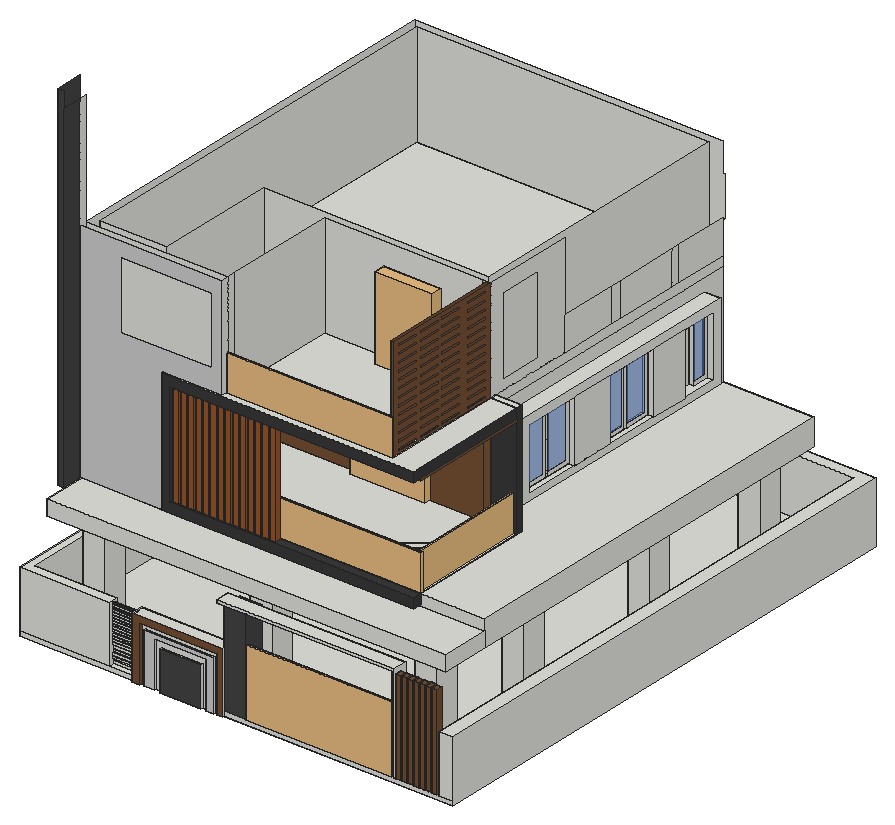
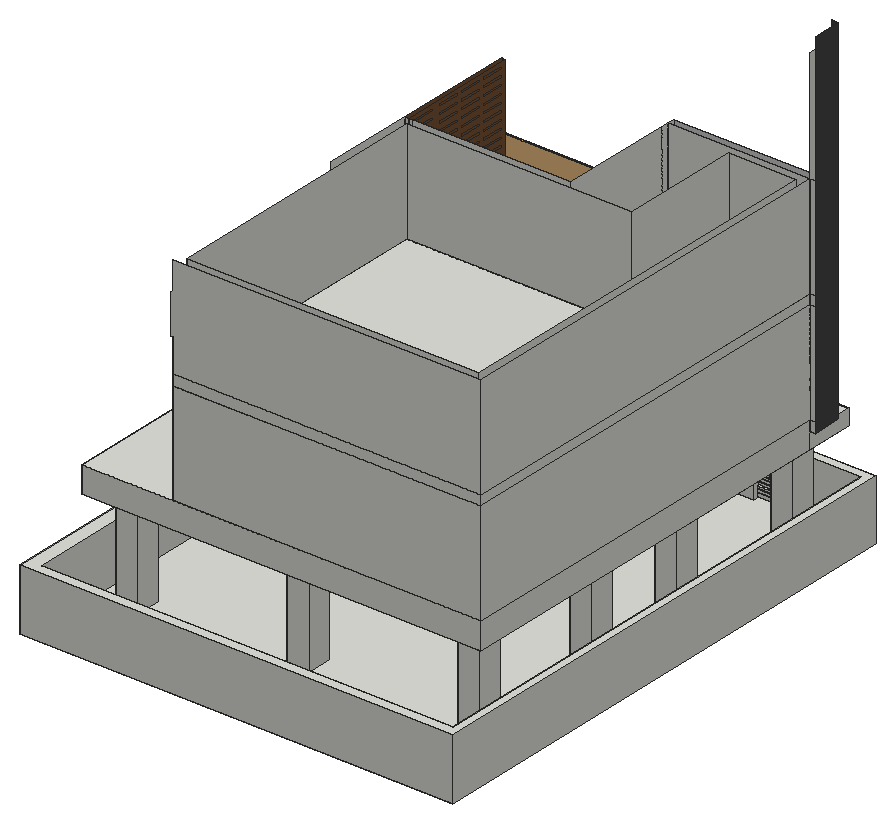
# SketchUp Ruby script. Lengths in inches.
U = 1.inch
M = Sketchup.active_model
def pt(a) = Geom::Point3d.new(a.map { |v| v * U })
def face(e, loops, mat)
  f = e.add_face(loops[0].map { |a| pt(a) })
  loops[1..].each { |l| e.add_face(l.map { |a| pt(a) }).erase! }
  f.material = f.back_material = mat if mat
  f
end
# faces: each face lists its corners as indices into pts; further lists are holes
def faces(e, pts, list, mat = nil) = list.each { |f| face(e, (f[0].is_a?(Array) ? f : [f]).map { |l| l.map { |i| pts[i] } }, mat) }
# xy, xz, yz: faces in a plane at the given z, y or x. An outline is a flat list of corners, or four numbers for a rectangle; further outlines are holes
def ring(l) = l.size == 4 ? [[l[0], l[1]], [l[2], l[1]], [l[2], l[3]], [l[0], l[3]]] : l.each_slice(2).to_a
def flat(e, list, mat, &to3) = list.each { |f| face(e, (f[0].is_a?(Array) ? f : [f]).map { |l| ring(l).map { |u, v| to3.(u, v) } }, mat) }
def xy(e, z, list, mat = nil) = flat(e, list, mat) { |x, y| [x, y, z] }
def xz(e, y, list, mat = nil) = flat(e, list, mat) { |x, z| [x, y, z] }
def yz(e, x, list, mat = nil) = flat(e, list, mat) { |y, z| [x, y, z] }
def lines(e, pts, list) = list.each { |a, b| e.add_line(pt(pts[a]), pt(pts[b])) }
# prism: a flat outline (further loops are holes) pulled along v
def prism(e, loops, v, mat = nil)
  f = face(e, loops, mat); d = Geom::Vector3d.new(v.map { |x| x * U })
  f.pushpull(f.normal.samedirection?(d) ? d.length : -d.length)
end
def box(e, o, s, mat = nil) = prism(e, [[o, [o[0] + s[0], o[1], o[2]], [o[0] + s[0], o[1] + s[1], o[2]], [o[0], o[1] + s[1], o[2]]]], [0, 0, s[2]], mat)
def at(x, y, z, deg = 0) = Geom::Transformation.translation(pt([x, y, z])) * Geom::Transformation.rotation(ORIGIN, Z_AXIS, deg.degrees)
def axes(o, x, y, z) = Geom::Transformation.new([*x, 0, *y, 0, *z, 0, *pt(o).to_a, 1])
def part(name) = M.definitions.add(name)
# library, detail: a bought-in or finely detailed component or shape, given as its bounding box
def library(name, o, s) = part(name).tap { |d| box(d.entities, o, s) }
def detail(e, o, s) = box(e.add_group.entities, o, s)
def put(e, d, t, mat = nil) = e.add_instance(d, t).tap { |i| i.material = mat if mat }
def group(e, t, mat = nil) = e.add_group.tap { |g| g.transformation = t; g.material = mat if mat }.entities
root = M.entities
M.materials.add("[Carrera Marble]").color = [207, 207, 207]
M.materials.add("[Color M07]").color = [58, 58, 58]
M.materials.add("[Granite Dark Gray]").color = [69, 68, 68]
M.materials.add("[Sandstone]").color = [118, 81, 52]
M.materials.add("[Translucent Glass Blue]").color = [100, 149, 237]
M.materials["[Translucent Glass Blue]"].alpha = 0.5
M.materials.add("[Wood Cherry Original]").color = [152, 86, 42]
c1 = part("Group\#1")
box(c1.entities,[0,-120,0],[26.125,120,28.5])
c2 = library("Modern Gate 1",[0,0,0],[118.11,1.97,78.74])
c3 = part("Group\#42")
box(c3.entities,[-2.625,0,0],[5.625,7.625,109.5625])
c4 = library("Wagner Glass Railing",[9.08,102.375,1.53],[2.51,145.5,42.05])
c5 = library("Glazed double door",[0,0,0],[62.99,7.48,78.74])
c6 = part("Group\#2")
box(c6.entities,[0,0,0],[7.1875,5.875,122.9375],"[Wood Cherry Original]")
c7 = part("Janela aluminio\#1")
xy(c7.entities,0,[[0,0,47.24,1.57],[23.62,1.57,47.24,2.76],[0,2.76,25.98,3.9375],[0,3.9375,47.24,5.91]])
xy(c7.entities,43.31,[[0,0,47.24,1.57],[23.62,1.57,47.24,2.76],[0,2.76,0,5.91,47.24,5.91,47.24,3.9375,25.98,3.9375,25.98,2.76],[25.98,2.76,47.24,3.9375]])
xz(c7.entities,1.57,[[0,0,23.62,0,23.62,41.34,21.26,41.34,21.26,1.97,1.97,1.97,1.97,41.34,23.62,41.34,23.62,43.31,0,43.31],[[23.62,0,47.24,43.31],[25.7,1.97,45.28,41.34]]])
xz(c7.entities,2.76,[[[0,0,23.62,43.31],[2.36,2.36,21.26,40.94]],[23.62,0,25.98,43.31]])
xz(c7.entities,2.76,[[2.36,2.36,21.26,40.94]],"[Translucent Glass Blue]")
xz(c7.entities,3.9375,[[25.98,0,25.98,2.36,44.88,2.36,44.88,40.94,25.98,40.94,25.98,43.31,47.24,43.31,47.24,0]])
xz(c7.entities,3.9375,[[25.98,2.36,44.88,40.94]],"[Translucent Glass Blue]")
yz(c7.entities,0,[[0,0,1.57,43.31],[2.76,0,5.91,43.31]])
yz(c7.entities,23.62,[[1.57,0,2.76,43.31]])
yz(c7.entities,25.98,[[2.76,0,3.9375,43.31]])
yz(c7.entities,47.24,[[0,0,1.57,43.31],[1.57,0,2.76,43.31],[3.9375,0,5.91,43.31]])
c8 = part("Group\#5")
prism(c8.entities,[[[0,0,131.51],[0,0,140.51],[8.96,0,140.51],[21.98,0,140.51],[21.98,0,0],[0,0,0]]],[0,-2.3125,0])
c9 = part("Group\#4")
box(c9.entities,[0,-480,0],[360,480,12])
c10 = library("test",[125.61,35.04,0],[12.99,66.93,96.46])
box(root,[18.76,18.85,-141.29],[466.13,57.13,17.95])
xy(root,-266.29,[[147.24,0,147.24,2.375,0,2.375,0,620.47,505.875,620.47,505.875,2.375,228.33,2.375,228.33,0,219.08,0,219.08,2.375,213.55,2.375,213.55,0,165.63,0,165.63,2.375,159.24,2.375,159.24,0],[133.09,0,142.08,2.375],[231.94,0,238.97,2.375]])
xy(root,-261.29,[[104.9,2.375,133.09,2.375,133.09,14.25,238.97,14.25,238.97,25.4375,264.34,25.4375,264.34,2.375,434.35,2.375,434.35,18.875,437.54,18.875,437.54,2.375,489.68,2.375,489.68,608.34,9.22,608.34,9.22,13.4,104.9,13.4],[238.97,2.375,264.34,25.4375]])
xy(root,-259.28,[[104.9,6.59,134.72,9.9]])
xy(root,-255.96,[[104.9,6.59,134.72,9.9]])
xy(root,-254.51,[[104.9,6.36,135.03,9.73]])
xy(root,-251.88,[[104.9,6.36,135.03,9.73]])
xy(root,-250.74,[[104.9,6.31,135.47,9.43]])
xy(root,-248.3,[[104.9,6.31,135.47,9.43]])
xy(root,-247.03,[[104.9,6.39,135.03,8.95]])
xy(root,-244.47,[[104.9,6.39,135.03,8.95]])
xy(root,-243.26,[[104.9,6.39,135.22,8.51]])
xy(root,-240.82,[[104.9,6.39,135.22,8.51]])
xy(root,-239.6,[[104.9,6.24,136.03,8.49]])
xy(root,-237.35,[[104.9,6.24,136.03,8.49]])
xy(root,-236.07,[[104.9,5.99,134.59,8.24]])
xy(root,-234.01,[[104.9,5.99,134.59,8.24]])
xy(root,-232.8,[[104.9,5.84,136.53,8.09]])
xy(root,-230.92,[[104.9,5.84,136.53,8.09]])
xy(root,-229.72,[[104.9,5.97,142.08,8.41]])
xy(root,-227.65,[[104.9,5.97,142.08,8.41]])
xy(root,-225.66,[[104.9,5.73,135.78,8.17]])
xy(root,-223.91,[[104.9,5.73,135.78,8.17]])
xy(root,-222.46,[[104.9,5.5625,133.34,7.875]])
xy(root,-221.03,[[165.63,0,213.55,2.375]])
xy(root,-220.78,[[104.9,5.5625,133.34,7.875]])
xy(root,-219.6,[[104.9,5.51,142.08,7.82]])
xy(root,-217.97,[[104.9,5.51,142.08,7.82]])
xy(root,-216.74,[[104.9,5.42,138.72,7.61]])
xy(root,-215.12,[[104.9,5.42,138.72,7.61]])
xy(root,-213.64,[[104.9,5.39,135.9,7.45]])
xy(root,-212.45,[[159.24,0,219.08,2.375]])
xy(root,-212.01,[[104.9,5.39,135.9,7.45]])
xy(root,-210.69,[[104.9,5.36,134.65,7.36]])
xy(root,-208.69,[[104.9,5.36,134.65,7.36]])
xy(root,-207.6,[[147.24,0,228.33,2.375]])
xy(root,-207.35,[[104.9,5.15,136.84,6.9]])
xy(root,-205.6,[[104.9,5.15,136.84,6.9]])
xy(root,-204.41,[[104.9,5.07,136.15,6.88]])
xy(root,-202.6,[[104.9,5.07,136.15,6.88]])
xy(root,-202.06,[[142.08,0,231.94,2.375]],"[Sandstone]")
xy(root,-201.5,[[104.9,5.28,134.97,6.85]])
xy(root,-199.93,[[104.9,5.28,134.97,6.85]])
xy(root,-198.85,[[104.9,5.125,134.53,6.875]])
xy(root,-197.28,[[104.9,5.125,134.53,6.875]])
xy(root,-196.375,[[104.9,5.06,135.09,6.75]])
xy(root,-194.875,[[104.9,5.06,135.09,6.75]])
xy(root,-194.79,[[133.09,0,238.97,14.25]])
xy(root,-194.41,[[0,2.375,104.9,2.375,104.9,13.4,9.22,13.4,9.22,608.34,489.68,608.34,489.68,2.375,505.875,2.375,505.875,620.47,0,620.47]])
xy(root,-150.83,[[229.85,2.375,238.97,18.875],[238.97,2.375,264.34,18.875],[264.34,2.375,434.35,18.875],[238.97,18.875,264.34,25.4375]])
xy(root,-147.41,[[229.85,2.375,437.54,18.875]])
xy(root,-122.04,[[11.76,42.54,18.76,75.98],[115.14,65.73,115.14,75.98,379.07,75.98,379.07,224.17,409.51,224.17,409.51,65.73],[18.76,67.23,115.14,75.98]])
xy(root,-110.04,[[[18.76,75.98,18.76,555.98,378.76,555.98,378.76,216.49,115.14,216.49,115.14,75.98],[27.76,84.98,106.14,84.98,106.14,225.49,369.76,225.49,369.76,546.98,27.76,546.98]],[115.14,75.98,378.76,216.49]])
xy(root,-110.04,[[124.1,65.73,409.51,75.98],[379.07,75.98,409.51,216.49]],"[Color M07]")
xy(root,-93.12,[[378.76,239.71,398.39,528.27]])
xy(root,-85.48,[[388.51,248.25,398.39,314.97],[384.07,366.08,398.39,430.88],[384.26,475.3,398.39,518.82]])
xy(root,-13.6,[[388.51,248.25,398.39,314.97],[384.07,366.08,398.39,430.88],[384.26,475.3,398.39,518.82]])
xy(root,-3.68,[[378.76,239.71,398.39,528.27]])
xy(root,9.96,[[[18.76,75.98,115.14,75.98,115.14,216.49,378.76,216.49,378.76,555.98,18.76,555.98],[27.76,84.98,27.76,546.98,369.76,546.98,369.76,225.49,106.14,225.49,106.14,84.98]],[137.11,75.98,378.76,216.49]])
xy(root,9.96,[[124.1,65.73,124.1,75.98,378.76,75.98,378.76,216.49,409.51,216.49,409.51,65.73]],"[Color M07]")
xy(root,21.96,[[115.14,65.73,409.51,65.73,409.51,216.49,378.76,216.49,378.76,75.98,184.57,75.98,184.57,67.23,115.14,67.23],[115.14,67.23,184.57,75.98],[[18.76,75.98,18.76,555.98,378.76,555.98,378.76,216.49,184.57,216.49,184.57,75.98],[27.76,84.98,106.14,84.98,106.14,225.49,369.76,225.49,369.76,546.98,27.76,546.98]],[184.57,75.98,374.26,75.98,374.26,216.49,369.76,216.49,369.76,84.98,184.57,84.98],[184.57,84.98,369.76,216.49],
  [379.07,216.49,409.51,224.17]])
xz(root,0,[[147.24,-266.29,159.24,-266.29,159.24,-212.45,219.08,-212.45,219.08,-266.29,228.33,-266.29,228.33,-207.6,147.24,-207.6]],"[Carrera Marble]")
xz(root,0,[[165.63,-266.29,213.55,-221.03]],"[Granite Dark Gray]")
xz(root,0,[[133.09,-266.29,142.08,-266.29,142.08,-202.06,231.94,-202.06,231.94,-266.29,238.97,-266.29,238.97,-194.79,133.09,-194.79]],"[Sandstone]")
xz(root,2.375,[[0,-266.29,133.09,-261.29],[142.08,-266.29,147.24,-266.29,147.24,-207.6,228.33,-207.6,228.33,-266.29,231.94,-266.29,231.94,-202.06,142.08,-202.06],[159.24,-266.29,165.63,-266.29,165.63,-221.03,213.55,-221.03,213.55,-266.29,219.08,-266.29,219.08,-212.45,159.24,-212.45],[238.97,-266.29,505.875,-266.29,505.875,-261.29,437.54,-261.29,437.54,-147.41,229.85,-147.41,229.85,-150.83,434.35,-150.83,434.35,-261.29,238.97,-261.29],[0,-261.29,104.9,-194.41],
  [489.68,-261.29,505.875,-194.41]])
xz(root,2.375,[[238.97,-261.29,264.34,-150.83]],"[Granite Dark Gray]")
xz(root,5.06,[[104.9,-196.375,135.09,-194.875]])
xz(root,5.07,[[104.9,-204.41,136.15,-202.6]])
xz(root,5.125,[[104.9,-198.85,134.53,-197.28]])
xz(root,5.15,[[104.9,-207.35,136.84,-205.6]])
xz(root,5.28,[[104.9,-201.5,134.97,-199.93]])
xz(root,5.36,[[104.9,-210.69,134.65,-208.69]])
xz(root,5.39,[[104.9,-213.64,135.9,-212.01]])
xz(root,5.42,[[104.9,-216.74,138.72,-215.12]])
xz(root,5.51,[[104.9,-219.6,142.08,-217.97]])
xz(root,5.5625,[[104.9,-222.46,133.34,-220.78]])
xz(root,5.73,[[104.9,-225.66,135.78,-223.91]])
xz(root,5.84,[[104.9,-232.8,136.53,-230.92]])
xz(root,5.97,[[104.9,-229.72,142.08,-227.65]])
xz(root,5.99,[[104.9,-236.07,134.59,-234.01]])
xz(root,6.24,[[104.9,-239.6,136.03,-237.35]])
xz(root,6.31,[[104.9,-250.74,135.47,-248.3]])
xz(root,6.36,[[104.9,-254.51,135.03,-251.88]])
xz(root,6.39,[[104.9,-247.03,135.03,-244.47],[104.9,-243.26,135.22,-240.82]])
xz(root,6.59,[[104.9,-259.28,134.72,-255.96]])
xz(root,6.75,[[104.9,-196.375,135.09,-194.875]])
xz(root,6.85,[[104.9,-201.5,134.97,-199.93]])
xz(root,6.875,[[104.9,-198.85,134.53,-197.28]])
xz(root,6.88,[[104.9,-204.41,136.15,-202.6]])
xz(root,6.9,[[104.9,-207.35,136.84,-205.6]])
xz(root,7.36,[[104.9,-210.69,134.65,-208.69]])
xz(root,7.45,[[104.9,-213.64,135.9,-212.01]])
xz(root,7.61,[[104.9,-216.74,138.72,-215.12]])
xz(root,7.82,[[104.9,-219.6,142.08,-217.97]])
xz(root,7.875,[[104.9,-222.46,133.34,-220.78]])
xz(root,8.09,[[104.9,-232.8,136.53,-230.92]])
xz(root,8.17,[[104.9,-225.66,135.78,-223.91]])
xz(root,8.24,[[104.9,-236.07,134.59,-234.01]])
xz(root,8.41,[[104.9,-229.72,142.08,-227.65]])
xz(root,8.49,[[104.9,-239.6,136.03,-237.35]])
xz(root,8.51,[[104.9,-243.26,135.22,-240.82]])
xz(root,8.95,[[104.9,-247.03,135.03,-244.47]])
xz(root,9.43,[[104.9,-250.74,135.47,-248.3]])
xz(root,9.73,[[104.9,-254.51,135.03,-251.88]])
xz(root,9.9,[[104.9,-259.28,134.72,-255.96]])
xz(root,13.4,[[9.22,-261.29,104.9,-194.41]])
xz(root,14.25,[[133.09,-261.29,238.97,-194.79]])
xz(root,18.875,[[434.35,-261.29,434.35,-150.83,229.85,-150.83,229.85,-147.41,437.54,-147.41,437.54,-261.29]])
xz(root,25.4375,[[238.97,-261.29,264.34,-150.83]])
xz(root,42.54,[[11.76,-122.04,18.76,293.28]],"[Granite Dark Gray]")
xz(root,65.73,[[115.14,-122.04,409.51,-122.04,409.51,-110.04,124.1,-110.04,124.1,9.96,409.51,9.96,409.51,21.96,115.14,21.96]],"[Color M07]")
xz(root,67.23,[[[18.76,-122.04,115.14,-122.04,115.14,21.96,184.57,21.96,184.57,141.96,18.76,141.96],[66.65,46.02,171.96,125.2]]],"[Carrera Marble]")
xz(root,75.98,[[11.76,-122.04,18.76,-110.04],[18.76,-122.04,115.14,-110.04],[115.14,-122.04,379.07,-110.04],[11.76,-110.04,18.76,9.96],[18.76,-110.04,115.14,9.96],
  [115.14,-110.04,124.1,9.96],[11.76,9.96,18.76,21.96],[18.76,9.96,115.14,21.96],[115.14,9.96,378.76,21.96],[11.76,21.96,18.76,141.96],
  [18.76,21.96,184.57,141.96]])
xz(root,75.98,[[374.26,21.96,378.76,141.96]],"[Sandstone]")
xz(root,84.98,[[27.76,-110.04,106.14,9.96],[27.76,21.96,106.14,141.96]])
xz(root,216.49,[[378.76,9.96,379.07,21.96],[379.07,9.96,409.51,21.96],[184.57,21.96,369.76,141.96],[369.76,21.96,374.26,141.96],[374.26,21.96,378.76,141.96]])
xz(root,216.49,[[379.07,-110.04,409.51,9.96]],"[Color M07]")
xz(root,216.49,[[115.14,-110.04,369.76,9.96],[369.76,-110.04,378.76,9.96]],"[Sandstone]")
xz(root,224.17,[[379.07,-122.04,409.51,21.96]])
xz(root,225.49,[[106.14,-110.04,369.76,9.96],[106.14,21.96,369.76,141.96]])
xz(root,239.71,[[378.76,-93.12,398.39,-3.68]])
xz(root,248.25,[[388.51,-85.48,398.39,-13.6]])
xz(root,314.97,[[388.51,-85.48,398.39,-13.6]])
xz(root,366.08,[[384.07,-85.48,398.39,-13.6]])
xz(root,430.88,[[384.07,-85.48,398.39,-13.6]])
xz(root,475.3,[[384.26,-85.48,398.39,-13.6]])
xz(root,518.82,[[384.26,-85.48,398.39,-13.6]])
xz(root,528.27,[[378.76,-93.12,398.39,-3.68]])
xz(root,546.98,[[27.76,-110.04,369.76,9.96],[27.76,21.96,369.76,141.96]])
xz(root,555.98,[[18.76,-110.04,378.76,9.96],[18.76,21.96,18.76,141.96,378.76,141.96,378.76,107.78,380.7,107.78,380.7,61.25,378.76,61.25,378.76,21.96]])
xz(root,608.34,[[9.22,-261.29,489.68,-194.41]])
xz(root,620.47,[[0,-266.29,505.875,-194.41]])
yz(root,0,[[2.375,-266.29,620.47,-194.41]])
yz(root,9.22,[[13.4,-261.29,608.34,-194.41]])
yz(root,11.76,[[42.54,-122.04,75.98,293.28]],"[Granite Dark Gray]")
yz(root,18.76,[[67.23,-122.04,75.98,273.96],[75.98,-110.04,555.98,9.96],[75.98,21.96,555.98,141.96]])
yz(root,18.76,[[42.54,-122.04,67.23,273.96]],"[Granite Dark Gray]")
yz(root,27.76,[[84.98,-110.04,546.98,9.96],[84.98,21.96,546.98,141.96]])
yz(root,104.9,[[[2.375,-261.29,13.4,-194.41],[6.59,-259.28,9.9,-255.96],[6.36,-254.51,9.73,-251.88],[6.31,-250.74,9.43,-248.3],[6.39,-247.03,8.95,-244.47],[6.39,-243.26,8.51,-240.82],[6.24,-239.6,8.49,-237.35],[5.97,-229.72,8.41,-227.65],[5.99,-236.07,8.24,-234.01],[5.73,-225.66,8.17,-223.91],[5.84,-232.8,8.09,-230.92],[5.36,-210.69,7.36,-208.69],[5.5625,-222.46,7.875,-220.78],[5.51,-219.6,7.82,-217.97],[5.42,-216.74,7.61,-215.12],[5.39,-213.64,7.45,-212.01],[5.07,-204.41,6.88,-202.6],[5.15,-207.35,6.9,-205.6],[5.125,-198.85,6.875,-197.28],[5.06,-196.375,6.75,-194.875],[5.28,-201.5,6.85,-199.93]]])
yz(root,106.14,[[84.98,-110.04,225.49,9.96],[84.98,21.96,225.49,141.96]])
yz(root,115.14,[[65.73,-122.04,67.23,21.96],[67.23,-122.04,75.98,21.96],[75.98,-110.04,84.98,9.96],[84.98,-110.04,216.49,9.96]])
yz(root,124.1,[[65.73,-110.04,75.98,9.96]],"[Color M07]")
yz(root,133.09,[[0,-266.29,0,-194.79,14.25,-194.79,14.25,-261.29,2.375,-261.29,2.375,-266.29]])
yz(root,133.34,[[5.5625,-222.46,7.875,-220.78]])
yz(root,134.53,[[5.125,-198.85,6.875,-197.28]])
yz(root,134.59,[[5.99,-236.07,8.24,-234.01]])
yz(root,134.65,[[5.36,-210.69,7.36,-208.69]])
yz(root,134.72,[[6.59,-259.28,9.9,-255.96]])
yz(root,134.97,[[5.28,-201.5,6.85,-199.93]])
yz(root,135.03,[[6.36,-254.51,9.73,-251.88],[6.39,-247.03,8.95,-244.47]])
yz(root,135.09,[[5.06,-196.375,6.75,-194.875]])
yz(root,135.22,[[6.39,-243.26,8.51,-240.82]])
yz(root,135.47,[[6.31,-250.74,9.43,-248.3]])
yz(root,135.78,[[5.73,-225.66,8.17,-223.91]])
yz(root,135.9,[[5.39,-213.64,7.45,-212.01]])
yz(root,136.03,[[6.24,-239.6,8.49,-237.35]])
yz(root,136.15,[[5.07,-204.41,6.88,-202.6]])
yz(root,136.53,[[5.84,-232.8,8.09,-230.92]])
yz(root,136.84,[[5.15,-207.35,6.9,-205.6]])
yz(root,138.72,[[5.42,-216.74,7.61,-215.12]])
yz(root,142.08,[[5.97,-229.72,8.41,-227.65],[5.51,-219.6,7.82,-217.97]])
yz(root,142.08,[[0,-266.29,2.375,-202.06]],"[Sandstone]")
yz(root,147.24,[[0,-266.29,2.375,-207.6]])
yz(root,159.24,[[0,-266.29,2.375,-212.45]])
yz(root,165.63,[[0,-266.29,2.375,-221.03]])
yz(root,184.57,[[67.23,21.96,75.98,141.96],[75.98,21.96,84.98,141.96],[84.98,21.96,216.49,141.96]])
yz(root,213.55,[[0,-266.29,2.375,-221.03]])
yz(root,219.08,[[0,-266.29,2.375,-212.45]])
yz(root,228.33,[[0,-266.29,2.375,-207.6]])
yz(root,229.85,[[2.375,-150.83,18.875,-147.41]])
yz(root,231.94,[[0,-266.29,2.375,-202.06]],"[Sandstone]")
yz(root,238.97,[[0,-266.29,2.375,-194.79],[2.375,-261.29,14.25,-194.79]])
yz(root,238.97,[[14.25,-261.29,14.25,-194.79,2.375,-194.79,2.375,-150.83,25.4375,-150.83,25.4375,-261.29]],"[Granite Dark Gray]")
yz(root,264.34,[[2.375,-261.29,25.4375,-150.83]],"[Granite Dark Gray]")
yz(root,369.76,[[225.49,-110.04,546.98,9.96],[225.49,21.96,546.98,141.96]])
yz(root,374.26,[[[75.98,21.96,216.49,141.96],[80.89,134.51,108.58,137.88],[80.89,125.35,108.58,128.73],[80.89,116.2,108.58,119.58],[80.89,107.05,108.58,110.42],[80.89,97.9,108.58,101.27],[112.7,134.51,140.39,137.88],[144.51,134.51,172.2,137.88],[182.01,134.51,209.7,137.88],[80.89,88.74,108.58,92.12],[80.89,79.59,108.58,82.97],[80.89,70.4375,108.58,73.8125],[80.89,61.29,108.58,64.66],[80.89,52.13,108.58,55.51],[112.7,125.35,140.39,128.73],[112.7,116.2,140.39,119.58],[112.7,107.05,140.39,110.42],[112.7,97.9,140.39,101.27],[112.7,88.74,140.39,92.12],[112.7,79.59,140.39,82.97],[112.7,70.4375,140.39,73.8125],[112.7,61.29,140.39,64.66],[112.7,52.13,140.39,55.51],[112.7,42.98,140.39,46.36],[112.7,33.83,140.39,37.2],[144.51,125.35,172.2,128.73],[144.51,116.2,172.2,119.58],[144.51,107.05,172.2,110.42],[144.51,97.9,172.2,101.27],[144.51,88.74,172.2,92.12],[144.51,79.59,172.2,82.97],[144.51,70.4375,172.2,73.8125],[144.51,61.29,172.2,64.66],[144.51,52.13,172.2,55.51],[144.51,33.83,172.2,37.2],[144.51,42.98,172.2,46.36],[182.01,61.29,209.7,64.66],[182.01,52.13,209.7,55.51],[182.01,42.98,209.7,46.36],[182.01,33.83,209.7,37.2],[182.01,24.68,209.7,28.05],[144.51,24.68,172.2,28.05],[112.7,24.68,140.39,28.05],[182.01,70.4375,209.7,73.8125],[182.01,79.59,209.7,82.97],[182.01,97.9,209.7,101.27],[182.01,107.05,209.7,110.42],[182.01,116.2,209.7,119.58],[182.01,125.35,209.7,128.73],[80.89,42.98,108.58,46.36],[80.89,33.83,108.58,37.2],[80.89,24.68,108.58,28.05],[182.01,88.74,209.7,92.12]]],"[Sandstone]")
yz(root,378.76,[[[216.49,-110.04,555.98,9.96],[239.71,-93.12,528.27,-3.68]],[80.89,6.37,108.58,9.75],[112.7,6.37,140.39,9.75],[144.51,6.37,172.2,9.75],[182.01,6.37,209.7,9.75],
  [[75.98,9.96,216.49,21.96],[182.01,15.52,209.7,18.9],[112.7,15.52,140.39,18.9],[144.51,15.52,172.2,18.9],[80.89,15.52,108.58,18.9]],[80.89,15.52,108.58,18.9],[112.7,15.52,140.39,18.9],[144.51,15.52,172.2,18.9],[182.01,15.52,209.7,18.9],
  [[216.49,21.96,324.38,141.96],[234.07,32.94,285.88,124.38]],[324.38,21.96,392.06,61.25],[392.06,21.96,406.38,61.25],[406.38,21.96,481.66,61.25],[481.66,21.96,490.64,61.25],
  [490.64,21.96,555.98,61.25]])
yz(root,378.76,[[[75.98,21.96,216.49,141.96],[80.89,134.51,108.58,137.88],[112.7,134.51,140.39,137.88],[144.51,134.51,172.2,137.88],[182.01,134.51,209.7,137.88],[182.01,125.35,209.7,128.73],[144.51,125.35,172.2,128.73],[112.7,125.35,140.39,128.73],[80.89,125.35,108.58,128.73],[182.01,116.2,209.7,119.58],[144.51,116.2,172.2,119.58],[112.7,116.2,140.39,119.58],[80.89,116.2,108.58,119.58],[182.01,107.05,209.7,110.42],[144.51,107.05,172.2,110.42],[112.7,107.05,140.39,110.42],[80.89,107.05,108.58,110.42],[182.01,97.9,209.7,101.27],[144.51,97.9,172.2,101.27],[112.7,97.9,140.39,101.27],[80.89,97.9,108.58,101.27],[182.01,88.74,209.7,92.12],[144.51,88.74,172.2,92.12],[112.7,88.74,140.39,92.12],[80.89,88.74,108.58,92.12],[182.01,79.59,209.7,82.97],[144.51,79.59,172.2,82.97],[112.7,79.59,140.39,82.97],[80.89,79.59,108.58,82.97],[182.01,70.4375,209.7,73.8125],[144.51,70.4375,172.2,73.8125],[112.7,70.4375,140.39,73.8125],[80.89,70.4375,108.58,73.8125],[182.01,61.29,209.7,64.66],[144.51,61.29,172.2,64.66],[112.7,61.29,140.39,64.66],[80.89,61.29,108.58,64.66],[182.01,52.13,209.7,55.51],[144.51,52.13,172.2,55.51],[112.7,52.13,140.39,55.51],[80.89,52.13,108.58,55.51],[182.01,42.98,209.7,46.36],[144.51,42.98,172.2,46.36],[112.7,42.98,140.39,46.36],[80.89,42.98,108.58,46.36],[182.01,33.83,209.7,37.2],[144.51,33.83,172.2,37.2],[112.7,33.83,140.39,37.2],[80.89,33.83,108.58,37.2],[182.01,24.68,209.7,28.05],[144.51,24.68,172.2,28.05],[112.7,24.68,140.39,28.05],[80.89,24.68,108.58,28.05]]],"[Sandstone]")
yz(root,379.07,[[75.98,-122.04,75.98,-110.04,216.49,-110.04,216.49,21.96,224.17,21.96,224.17,-122.04]])
yz(root,384.07,[[366.08,-85.48,430.88,-13.6]])
yz(root,384.26,[[475.3,-85.48,518.82,-13.6]])
yz(root,388.51,[[248.25,-85.48,314.97,-13.6]])
yz(root,398.39,[[[239.71,-93.12,528.27,-3.68],[248.25,-85.48,518.82,-13.6]],[314.97,-85.48,366.08,-13.6],[430.88,-85.48,475.3,-13.6]])
yz(root,409.51,[[65.73,-122.04,224.17,-122.04,224.17,21.96,216.49,21.96,216.49,-110.04,65.73,-110.04],[65.73,9.96,216.49,21.96]],"[Color M07]")
yz(root,434.35,[[2.375,-261.29,18.875,-150.83]])
yz(root,437.54,[[2.375,-261.29,18.875,-147.41]])
yz(root,489.68,[[2.375,-261.29,608.34,-194.41]])
yz(root,505.875,[[2.375,-266.29,620.47,-194.41]])
p = [[369.76,84.98,-110.04],[369.76,216.49,-110.04],[219.08,2.375,-212.45],[228.33,2.375,-212.45]]
lines(root,p,[[0,1],[2,3]])
put(root,c1,axes([439.11,59.125,-141.29],[1,0,0],[0,0,1],[0,-1,0]))
put(root,c2,axes([264.34,4.34,-182.55],[1.43939,0,0],[0,-1,0],[0,0,-1]))
put(root,c1,axes([51.04,59.125,-141.29],[1,0,0],[0,0,1],[0,-1,0]))
put(root,c1,axes([246.67,59.125,-141.29],[1,0,0],[0,0,1],[0,-1,0]))
put(root,c3,at(484.11,2.375,-261.29),"[Sandstone]")
put(root,c3,at(477.5,10.38,-261.29,-180),"[Sandstone]")
put(root,c3,at(469.82,2.74,-261.29),"[Sandstone]")
put(root,c3,at(463.46,9.95,-261.29,-180),"[Sandstone]")
put(root,c3,at(455.9,2.26,-261.29),"[Sandstone]")
put(root,c3,at(448.79,2.26,-261.29),"[Sandstone]")
put(root,c3,at(442.05,10,-261.29,-180),"[Sandstone]")
put(root,c1,axes([439.11,185.875,-141.29],[1,0,0],[0,0,1],[0,-1,0]))
put(root,c1,axes([51.04,228.625,-141.29],[1,0,0],[0,0,1],[0,-1,0]))
put(root,c1,axes([439.11,369.4375,-141.29],[1,0,0],[0,0,1],[0,-1,0]))
put(root,c1,axes([51.04,353.1875,-141.29],[1,0,0],[0,0,1],[0,-1,0]))
put(root,c1,axes([51.04,517,-141.29],[1,0,0],[0,0,1],[0,-1,0]))
put(root,c1,axes([250.11,517,-141.29],[1,0,0],[0,0,1],[0,-1,0]))
put(root,c1,axes([439.11,531.3125,-141.29],[1,0,0],[0,0,1],[0,-1,0]))
g1 = group(root,at(18.76,555.98,-122.04))
box(g1,[0,-480,-19.25],[466.125,480,31.25])
put(root,c4,axes([395.38,-18.3125,-111.57],[1,0,0],[0,0.93845,0],[0,0,1]))
put(root,c5,axes([220.89,209.01,-110.04],[1.38,0,0],[0,1,0],[0,0,1.3]))
put(root,c6,at(126.58,68.11,-110.04),"[Wood Cherry Original]")
put(root,c6,at(135.27,68.11,-110.04),"[Wood Cherry Original]")
put(root,c6,at(143.95,68.11,-110.04),"[Wood Cherry Original]")
put(root,c6,at(152.64,68.11,-110.04),"[Wood Cherry Original]")
put(root,c6,at(161.33,68.11,-110.04),"[Wood Cherry Original]")
put(root,c6,at(170.02,68.11,-110.04),"[Wood Cherry Original]")
put(root,c6,at(178.7,68.11,-110.04),"[Wood Cherry Original]")
put(root,c6,at(187.39,68.11,-110.04),"[Wood Cherry Original]")
put(root,c6,at(196.08,68.11,-110.04),"[Wood Cherry Original]")
put(root,c6,at(204.7,68.11,-110.04),"[Wood Cherry Original]")
put(root,c6,at(213.33,68.11,-110.04),"[Wood Cherry Original]")
put(root,c6,at(221.95,68.11,-110.04),"[Wood Cherry Original]")
put(root,c6,at(230.77,68.11,-110.04),"[Wood Cherry Original]")
put(root,c6,at(239.27,68.11,-110.04),"[Wood Cherry Original]")
put(root,c4,axes([525.25,66.9,-111.57],[0,1,0],[-1.13058,0,0],[0,0,1]))
put(root,c7,axes([372.22,475.3,-13.6],[0,0.92112,0],[4.43,0,0],[0,0,-1.66716]))
put(root,c7,axes([389.7,248.65,-13.6],[0,1.40366,0],[0.33333,0,0],[0,0,-1.65966]))
put(root,c7,axes([389.7,363.78,-13.6],[0,1.40366,0],[0.33333,0,0],[0,0,-1.65966]))
put(root,c8,axes([388.07,216.49,9.96],[1,0,0],[0,0,1],[0,-1,0]),"[Sandstone]")
put(root,c8,axes([363.26,216.49,9.96],[1,0,0],[0,0,1],[0,-1,0]),"[Sandstone]")
put(root,c8,axes([338.45,216.49,9.96],[1,0,0],[0,0,1],[0,-1,0]),"[Sandstone]")
put(root,c8,axes([313.64,216.49,9.96],[1,0,0],[0,0,1],[0,-1,0]),"[Sandstone]")
put(root,c8,axes([288.82,216.49,9.96],[1,0,0],[0,0,1],[0,-1,0]),"[Sandstone]")
put(root,c8,axes([264.01,216.49,9.96],[1,0,0],[0,0,1],[0,-1,0]),"[Sandstone]")
put(root,c8,axes([239.2,216.49,9.96],[1,0,0],[0,0,1],[0,-1,0]),"[Sandstone]")
put(root,c8,axes([214.39,216.49,9.96],[1,0,0],[0,0,1],[0,-1,0]),"[Sandstone]")
put(root,c8,axes([189.57,216.49,9.96],[1,0,0],[0,0,1],[0,-1,0]),"[Sandstone]")
put(root,c8,axes([164.76,216.49,9.96],[1,0,0],[0,0,1],[0,-1,0]),"[Sandstone]")
put(root,c8,axes([139.95,216.49,9.96],[1,0,0],[0,0,1],[0,-1,0]),"[Sandstone]")
put(root,c8,axes([115.14,216.49,9.96],[1,0,0],[0,0,1],[0,-1,0]),"[Sandstone]")
put(root,c9,at(18.76,555.98,9.96))
put(root,c10,axes([221.64,74.35,118.42],[0,1,0],[1,0,0],[0,0,-1]))
put(root,c4,axes([515.39,64.38,20.43],[0,1,0],[-1.33462,0,0],[0,0,1]))
